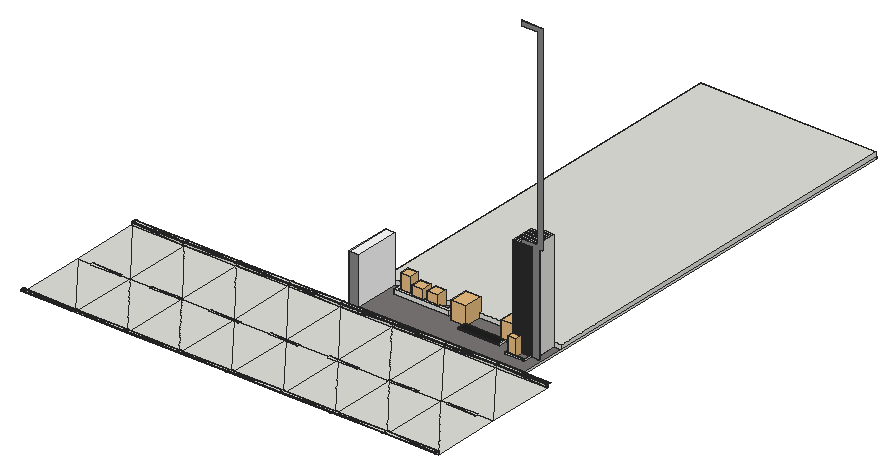
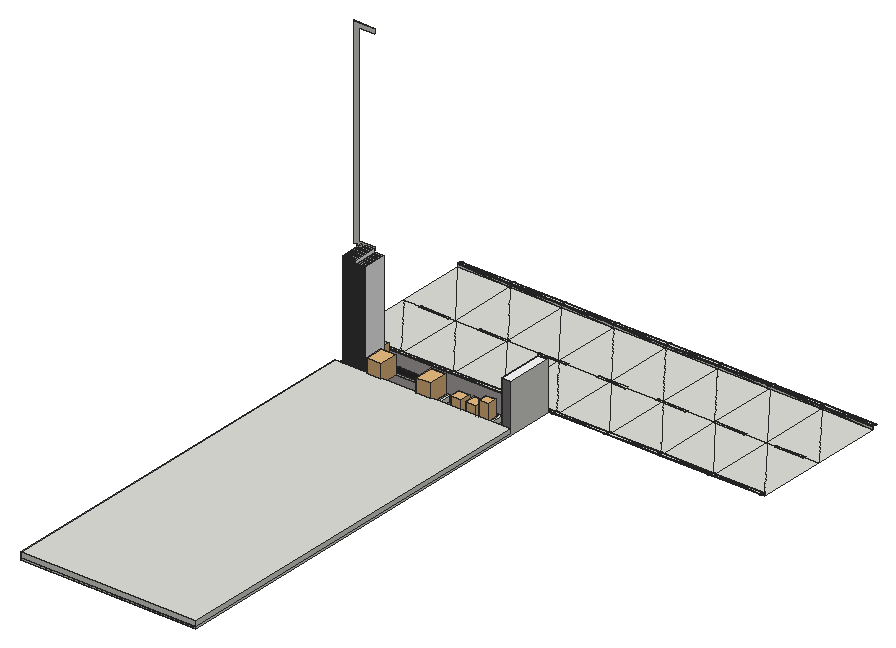
# SketchUp Ruby script. Lengths in inches.
U = 1.inch
M = Sketchup.active_model
def pt(a) = Geom::Point3d.new(a.map { |v| v * U })
def face(e, loops, mat)
  f = e.add_face(loops[0].map { |a| pt(a) })
  loops[1..].each { |l| e.add_face(l.map { |a| pt(a) }).erase! }
  f.material = f.back_material = mat if mat
  f
end
# faces: each face lists its corners as indices into pts; further lists are holes
def faces(e, pts, list, mat = nil) = list.each { |f| face(e, (f[0].is_a?(Array) ? f : [f]).map { |l| l.map { |i| pts[i] } }, mat) }
# xy, xz, yz: faces in a plane at the given z, y or x. An outline is a flat list of corners, or four numbers for a rectangle; further outlines are holes
def ring(l) = l.size == 4 ? [[l[0], l[1]], [l[2], l[1]], [l[2], l[3]], [l[0], l[3]]] : l.each_slice(2).to_a
def flat(e, list, mat, &to3) = list.each { |f| face(e, (f[0].is_a?(Array) ? f : [f]).map { |l| ring(l).map { |u, v| to3.(u, v) } }, mat) }
def xy(e, z, list, mat = nil) = flat(e, list, mat) { |x, y| [x, y, z] }
def xz(e, y, list, mat = nil) = flat(e, list, mat) { |x, z| [x, y, z] }
def yz(e, x, list, mat = nil) = flat(e, list, mat) { |y, z| [x, y, z] }
def lines(e, pts, list) = list.each { |a, b| e.add_line(pt(pts[a]), pt(pts[b])) }
# prism: a flat outline (further loops are holes) pulled along v
def prism(e, loops, v, mat = nil)
  f = face(e, loops, mat); d = Geom::Vector3d.new(v.map { |x| x * U })
  f.pushpull(f.normal.samedirection?(d) ? d.length : -d.length)
end
def box(e, o, s, mat = nil) = prism(e, [[o, [o[0] + s[0], o[1], o[2]], [o[0] + s[0], o[1] + s[1], o[2]], [o[0], o[1] + s[1], o[2]]]], [0, 0, s[2]], mat)
def at(x, y, z, deg = 0) = Geom::Transformation.translation(pt([x, y, z])) * Geom::Transformation.rotation(ORIGIN, Z_AXIS, deg.degrees)
def axes(o, x, y, z) = Geom::Transformation.new([*x, 0, *y, 0, *z, 0, *pt(o).to_a, 1])
def part(name) = M.definitions.add(name)
# library, detail: a bought-in or finely detailed component or shape, given as its bounding box
def library(name, o, s) = part(name).tap { |d| box(d.entities, o, s) }
def detail(e, o, s) = box(e.add_group.entities, o, s)
def put(e, d, t, mat = nil) = e.add_instance(d, t).tap { |i| i.material = mat if mat }
def group(e, t, mat = nil) = e.add_group.tap { |g| g.transformation = t; g.material = mat if mat }.entities
root = M.entities
M.materials.add("Marble White 602 38.29cm").color = [255, 255, 255]
M.materials.add("T8500 Silicone plaster D1 27.81cm").color = [255, 255, 255]
M.materials.add("Tiles B 130cm").color = [122, 119, 118]
M.materials.add("Tiles Marble Black 01 160cm").color = [32, 32, 32]
M.materials.add("Wall Paint Bumpy 01 Gray 100cm").color = [135, 135, 135]
M.materials.add("Wood Amboyan 13.2cm").color = [255, 255, 255]
c1 = library("Potted Plant 02",[-16.98,-19.78,0],[30.04,38.68,37.52])
c2 = library("Indoor Plant 004",[-26.75,-21.09,0],[44.44,41.03,87.36])
c3 = library("Potted Plant 50-12",[-6.11,-5.26,0],[11.24,10.56,13.41])
c4 = library("Sedum Plant 66-24",[-7.97,-7.95,0.04],[16.42,16.31,19.57])
c5 = library("Potted Plant 13",[-10,-7.28,0],[18.93,15.17,39.22])
c6 = part("Vertical panel \#2")
box(c6.entities,[0,-6.5625,0],[1.16,30,129.34],"Wood Amboyan 13.2cm")
c7 = part("Vertical panel \#1")
xy(c7.entities,0,[[0,-6.5625,1.16,23.4375]])
xy(c7.entities,125.9,[[0,-6.5625,1.16,23.4375]])
xz(c7.entities,-6.5625,[[0,0,1.16,125.9]],"Wood Amboyan 13.2cm")
xz(c7.entities,23.4375,[[0,0,1.16,125.9]])
yz(c7.entities,0,[[-6.5625,0,23.4375,125.9]])
yz(c7.entities,1.16,[[-6.5625,0,23.4375,125.9]])
c8 = part("Vertical panel \#3")
box(c8.entities,[0,-6.6875,0],[1.16,30.125,129.71],"Wood Amboyan 13.2cm")
c9 = part("Vertical panel \#4")
box(c9.entities,[0,-6.5625,0],[1.16,30,129.34],"Wood Amboyan 13.2cm")
c10 = part("Vertical panel \#5")
box(c10.entities,[0,-6.6875,0],[1.16,30.125,129.21],"Wood Amboyan 13.2cm")
c11 = part("Vertical panel \#6")
xy(c11.entities,0,[[0,0,1.16,23.4375]])
xy(c11.entities,129.21,[[0,0,1.16,23.4375]])
xz(c11.entities,0,[[0,0,1.16,129.21]],"Wood Amboyan 13.2cm")
xz(c11.entities,23.4375,[[0,0,1.16,129.21]])
yz(c11.entities,0,[[0,0,23.4375,129.21]])
yz(c11.entities,1.16,[[0,0,23.4375,129.21]])
c12 = part("Vertical panel \#7")
box(c12.entities,[0,-6.5625,0],[1.16,30,129.21])
c13 = part("Vertical panel assembly")
put(c13.entities,c9,at(0,0,0),"Wood Amboyan 13.2cm")
put(c13.entities,c10,at(2.58,0,0))
put(c13.entities,c11,at(5.16,0,0))
put(c13.entities,c12,at(7.75,0,0))
c14 = part("Component\#12")
xy(c14.entities,0,[[0,0,53.8125,10.8125]])
xy(c14.entities,1.8125,[[0,-0.5,2,0],[2,-0.5,51.8125,0],[51.8125,-0.5,53.8125,0]])
xy(c14.entities,2.125,[[51.8125,-0.5,53.8125,10.8125]])
xy(c14.entities,2.125,[[0,-0.5,2,10.8125]],"Marble White 602 38.29cm")
xy(c14.entities,2.125,[[2,-0.5,51.8125,10.8125]],"Tiles Marble Black 01 160cm")
xz(c14.entities,-0.5,[[0,1.8125,53.8125,2.125]],"Marble White 602 38.29cm")
xz(c14.entities,0,[[0,0,53.8125,1.8125]],"Tiles Marble Black 01 160cm")
xz(c14.entities,10.8125,[[0,0,53.8125,2.125]])
yz(c14.entities,0,[[0,0,0,1.8125,-0.5,1.8125,-0.5,2.125,10.8125,2.125,10.8125,0]])
yz(c14.entities,53.8125,[[0,0,10.8125,0,10.8125,2.125,-0.5,2.125,-0.5,1.8125,0,1.8125]])
xy(root,-10.11,[[0,4.875,66.91,4.875,0,92.46],[66.91,4.875,66.91,92.46,0,92.46],[133.82,4.875,133.82,92.46,66.91,92.46],[66.91,4.875,133.82,4.875,66.91,92.46],[133.82,4.875,200.73,4.875,133.82,92.46],
  [200.73,4.875,200.73,92.46,133.82,92.46],[200.73,4.875,267.64,4.875,200.73,92.46],[267.64,4.875,267.64,92.46,200.73,92.46],[267.64,4.875,334.55,4.875,267.64,92.46],[334.55,4.875,334.55,92.46,267.64,92.46],
  [334.55,4.875,401.46,4.875,334.55,92.46],[401.46,4.875,401.46,92.46,334.55,92.46],[401.46,4.875,468.37,4.875,401.46,92.46],[468.37,4.875,468.37,92.46,401.46,92.46],[468.37,4.875,535.28,4.875,468.37,92.46],
  [535.28,4.875,535.28,92.46,468.37,92.46],[0,92.46,66.91,92.46,0,180.06],[66.91,92.46,66.91,180.06,0,180.06],[133.82,92.46,133.82,180.06,66.91,180.06],[66.91,92.46,133.82,92.46,66.91,180.06],
  [133.82,92.46,200.73,92.46,133.82,180.06],[200.73,92.46,200.73,180.06,133.82,180.06],[200.73,92.46,267.64,92.46,200.73,180.06],[267.64,92.46,267.64,180.06,200.73,180.06],[267.64,92.46,334.55,92.46,267.64,180.06],
  [334.55,92.46,334.55,180.06,267.64,180.06],[334.55,92.46,401.46,92.46,334.55,180.06],[401.46,92.46,401.46,180.06,334.55,180.06],[401.46,92.46,468.37,92.46,401.46,180.06],[468.37,92.46,468.37,180.06,401.46,180.06],
  [468.37,92.46,535.28,92.46,468.37,180.06],[535.28,92.46,535.28,180.06,468.37,180.06]])
xy(root,-10.1,[[17.9,90.98,56.09,90.98,17.9,93.94],[56.09,90.98,56.09,93.94,17.9,93.94],[132.47,90.98,132.47,93.94,94.28,93.94],[94.28,90.98,132.47,90.98,94.28,93.94],[170.67,90.98,208.86,90.98,170.67,93.94],
  [208.86,90.98,208.86,93.94,170.67,93.94],[247.05,90.98,285.24,90.98,247.05,93.94],[285.24,90.98,285.24,93.94,247.05,93.94],[323.43,90.98,361.62,90.98,323.43,93.94],[361.62,90.98,361.62,93.94,323.43,93.94],
  [399.8125,90.98,438.01,90.98,399.8125,93.94],[438.01,90.98,438.01,93.94,399.8125,93.94],[476.2,90.98,514.39,90.98,476.2,93.94],[514.39,90.98,514.39,93.94,476.2,93.94]])
xy(root,-8.375,[[275.19,185.76,501.69,751.57]])
xy(root,-6,[[0,0.15,0.21,0.15,0,0.34],[0.21,0.15,0.21,0.34,0,0.34],[0.21,0.15,66.91,0.15,0.21,0.34],[66.91,0.15,66.91,0.34,0.21,0.34],[66.91,0.15,133.82,0.15,133.82,0.34],
  [66.91,0.15,133.82,0.34,66.91,0.34],[133.82,0.15,200.73,0.15,200.73,0.34],[133.82,0.15,200.73,0.34,133.82,0.34],[200.73,0.15,267.64,0.15,200.73,0.34],[267.64,0.15,267.64,0.34,200.73,0.34],
  [267.64,0.15,334.55,0.15,334.55,0.34],[267.64,0.15,334.55,0.34,267.64,0.34],[334.55,0.15,401.46,0.15,401.46,0.34],[334.55,0.15,401.46,0.34,334.55,0.34],[401.46,0.15,468.37,0.15,468.37,0.34],
  [401.46,0.15,468.37,0.34,401.46,0.34],[468.37,0.15,535.06,0.15,468.37,0.34],[535.06,0.15,535.06,0.34,468.37,0.34],[535.06,0.15,535.28,0.15,535.06,0.34],[535.28,0.15,535.28,0.34,535.06,0.34],
  [0,0.34,0.21,0.34,0,4.1],[0.21,0.34,0.21,4.1,0,4.1],[0.21,0.34,66.91,0.34,0.21,4.1],[66.91,0.34,66.91,4.1,0.21,4.1],[66.91,0.34,133.82,0.34,133.82,4.1],
  [66.91,0.34,133.82,4.1,66.91,4.1],[133.82,0.34,200.73,0.34,200.73,4.1],[133.82,0.34,200.73,4.1,133.82,4.1],[200.73,0.34,267.64,0.34,267.64,4.1],[200.73,0.34,267.64,4.1,200.73,4.1],
  [267.64,0.34,334.55,0.34,334.55,4.1],[267.64,0.34,334.55,4.1,267.64,4.1],[334.55,0.34,401.46,0.34,401.46,4.1],[334.55,0.34,401.46,4.1,334.55,4.1],[401.46,0.34,468.37,0.34,468.37,4.1],
  [401.46,0.34,468.37,4.1,401.46,4.1],[468.37,0.34,535.06,0.34,468.37,4.1],[535.06,0.34,535.06,4.1,468.37,4.1],[535.06,0.34,535.28,0.34,535.06,4.1],[535.28,0.34,535.28,4.1,535.06,4.1],
  [0,4.1,0.21,4.1,0,4.52],[0.21,4.1,0.21,4.52,0,4.52],[0.21,4.1,66.91,4.1,0.21,4.52],[66.91,4.1,66.91,4.52,0.21,4.52],[133.82,4.1,133.82,4.52,66.91,4.52],
  [66.91,4.1,133.82,4.1,66.91,4.52],[133.82,4.1,200.73,4.1,133.82,4.52],[200.73,4.1,200.73,4.52,133.82,4.52],[200.73,4.1,267.64,4.1,267.64,4.52],[200.73,4.1,267.64,4.52,200.73,4.52],
  [267.64,4.1,334.55,4.1,267.64,4.52],[334.55,4.1,334.55,4.52,267.64,4.52],[334.55,4.1,401.46,4.1,334.55,4.52],[401.46,4.1,401.46,4.52,334.55,4.52],[401.46,4.1,468.37,4.1,401.46,4.52],
  [468.37,4.1,468.37,4.52,401.46,4.52],[468.37,4.1,535.06,4.1,468.37,4.52],[535.06,4.1,535.06,4.52,468.37,4.52],[535.06,4.1,535.28,4.1,535.06,4.52],[535.28,4.1,535.28,4.52,535.06,4.52],
  [0,180.41,0.23,180.41,0,180.66],[0.23,180.41,0.23,180.66,0,180.66],[0.23,180.41,66.91,180.41,0.23,180.66],[66.91,180.41,66.91,180.66,0.23,180.66],[66.91,180.41,133.82,180.41,133.82,180.66],
  [66.91,180.41,133.82,180.66,66.91,180.66],[133.82,180.41,200.73,180.41,200.73,180.66],[133.82,180.41,200.73,180.66,133.82,180.66],[200.73,180.41,267.64,180.41,200.73,180.66],[267.64,180.41,267.64,180.66,200.73,180.66],
  [267.64,180.41,334.55,180.41,334.55,180.66],[267.64,180.41,334.55,180.66,267.64,180.66],[334.55,180.41,401.46,180.41,401.46,180.66],[334.55,180.41,401.46,180.66,334.55,180.66],[401.46,180.41,468.37,180.41,468.37,180.66],
  [401.46,180.41,468.37,180.66,401.46,180.66],[468.37,180.41,535.01,180.41,468.37,180.66],[535.01,180.41,535.01,180.66,468.37,180.66],[535.01,180.41,535.28,180.41,535.01,180.66],[535.28,180.41,535.28,180.66,535.01,180.66],
  [0,180.66,0.23,180.66,0,184.49],[0.23,180.66,0.23,184.49,0,184.49],[0.23,180.66,66.91,180.66,0.23,184.49],[66.91,180.66,66.91,184.49,0.23,184.49],[66.91,180.66,133.82,180.66,133.82,184.49],
  [66.91,180.66,133.82,184.49,66.91,184.49],[133.82,180.66,200.73,180.66,200.73,184.49],[133.82,180.66,200.73,184.49,133.82,184.49],[200.73,180.66,267.64,180.66,267.64,184.49],[200.73,180.66,267.64,184.49,200.73,184.49],
  [267.64,180.66,334.55,180.66,334.55,184.49],[267.64,180.66,334.55,184.49,267.64,184.49],[334.55,180.66,401.46,180.66,401.46,184.49],[334.55,180.66,401.46,184.49,334.55,184.49],[401.46,180.66,468.37,180.66,468.37,184.49],
  [401.46,180.66,468.37,184.49,401.46,184.49],[468.37,180.66,535.01,180.66,468.37,184.49],[535.01,180.66,535.01,184.49,468.37,184.49],[535.01,180.66,535.28,180.66,535.01,184.49],[535.28,180.66,535.28,184.49,535.01,184.49],
  [0,184.49,0.23,184.49,0,184.78],[0.23,184.49,0.23,184.78,0,184.78],[0.23,184.49,66.91,184.49,0.23,184.78],[66.91,184.49,66.91,184.78,0.23,184.78],[133.82,184.49,133.82,184.78,66.91,184.78],
  [66.91,184.49,133.82,184.49,66.91,184.78],[133.82,184.49,200.73,184.49,133.82,184.78],[200.73,184.49,200.73,184.78,133.82,184.78],[200.73,184.49,267.64,184.49,267.64,184.78],[200.73,184.49,267.64,184.78,200.73,184.78],
  [267.64,184.49,334.55,184.49,267.64,184.78],[334.55,184.49,334.55,184.78,267.64,184.78],[334.55,184.49,401.46,184.49,334.55,184.78],[401.46,184.49,401.46,184.78,334.55,184.78],[401.46,184.49,468.37,184.49,401.46,184.78],
  [468.37,184.49,468.37,184.78,401.46,184.78],[468.37,184.49,535.01,184.49,468.37,184.78],[535.01,184.49,535.01,184.78,468.37,184.78],[535.01,184.49,535.28,184.49,535.01,184.78],[535.28,184.49,535.28,184.78,535.01,184.78]])
xy(root,-6,[[[287.19,185.76,501.69,185.76,501.69,751.57,275.19,751.57,275.19,244.57,287.19,244.57],[297.97,228.57,297.97,244.57,301.97,244.57,301.97,232.57,365.1,232.57,365.1,244.57,369.1,244.57,369.1,228.57]]],"Tiles B 130cm")
xy(root,-5.9,[[462.69,202.57,462.69,214.57,463.69,214.57,463.69,203.57,486.92,203.57,486.92,213.79,487.92,213.79,487.92,202.57],[487.92,213.79,497.86,214.57],[475.6,214.57,476.76,244.57]])
xy(root,-0.4375,[[297.97,228.57,369.1,228.57,369.1,244.57,365.1,244.57,365.1,232.57,301.97,232.57,301.97,244.57,297.97,244.57]])
xy(root,54,[[275.19,185.76,287.19,244.57]],"T8500 Silicone plaster D1 27.81cm")
xz(root,0,[[0,-6.69,0.21,-6.69,0,-6.26],[0.21,-6.69,0.21,-6.26,0,-6.26],[0.21,-6.69,66.91,-6.69,0.21,-6.26],[66.91,-6.69,66.91,-6.26,0.21,-6.26],[66.91,-6.69,133.82,-6.26,66.91,-6.26],
  [66.91,-6.69,133.82,-6.69,133.82,-6.26],[133.82,-6.69,200.73,-6.26,133.82,-6.26],[133.82,-6.69,200.73,-6.69,200.73,-6.26],[200.73,-6.69,267.64,-6.26,200.73,-6.26],[200.73,-6.69,267.64,-6.69,267.64,-6.26],
  [267.64,-6.69,334.55,-6.26,267.64,-6.26],[267.64,-6.69,334.55,-6.69,334.55,-6.26],[334.55,-6.69,401.46,-6.26,334.55,-6.26],[334.55,-6.69,401.46,-6.69,401.46,-6.26],[401.46,-6.69,468.37,-6.26,401.46,-6.26],
  [401.46,-6.69,468.37,-6.69,468.37,-6.26],[468.37,-6.69,535.06,-6.69,468.37,-6.26],[535.06,-6.69,535.06,-6.26,468.37,-6.26],[535.06,-6.69,535.28,-6.69,535.06,-6.26],[535.28,-6.69,535.28,-6.26,535.06,-6.26]])
xz(root,4.875,[[0,-10.11,0,-6.93,0.21,-6.93],[0,-10.11,0.21,-6.93,0.21,-10.11],[0.21,-10.11,0.21,-6.93,66.91,-6.93],[0.21,-10.11,66.91,-6.93,66.91,-10.11],[66.91,-10.11,133.82,-6.93,133.82,-10.11],
  [66.91,-10.11,66.91,-6.93,133.82,-6.93],[133.82,-10.11,133.82,-6.93,200.73,-6.93],[133.82,-10.11,200.73,-6.93,200.73,-10.11],[200.73,-10.11,200.73,-6.93,267.64,-10.11],[267.64,-10.11,200.73,-6.93,267.64,-6.93],
  [267.64,-10.11,267.64,-6.93,334.55,-6.93],[267.64,-10.11,334.55,-6.93,334.55,-10.11],[334.55,-10.11,334.55,-6.93,401.46,-6.93],[334.55,-10.11,401.46,-6.93,401.46,-10.11],[401.46,-10.11,401.46,-6.93,468.37,-6.93],
  [401.46,-10.11,468.37,-6.93,468.37,-10.11],[468.37,-10.11,468.37,-6.93,535.06,-6.93],[468.37,-10.11,535.06,-6.93,535.06,-10.11],[535.06,-10.11,535.06,-6.93,535.28,-6.93],[535.06,-10.11,535.28,-6.93,535.28,-10.11],
  [0,-6.93,0,-6.49,0.21,-6.49],[0,-6.93,0.21,-6.49,0.21,-6.93],[0.21,-6.93,0.21,-6.49,66.91,-6.49],[0.21,-6.93,66.91,-6.49,66.91,-6.93],[133.82,-6.93,66.91,-6.49,133.82,-6.49],
  [66.91,-6.93,66.91,-6.49,133.82,-6.93],[133.82,-6.93,133.82,-6.49,200.73,-6.93],[200.73,-6.93,133.82,-6.49,200.73,-6.49],[200.73,-6.93,200.73,-6.49,267.64,-6.49],[200.73,-6.93,267.64,-6.49,267.64,-6.93],
  [267.64,-6.93,267.64,-6.49,334.55,-6.93],[334.55,-6.93,267.64,-6.49,334.55,-6.49],[334.55,-6.93,334.55,-6.49,401.46,-6.93],[401.46,-6.93,334.55,-6.49,401.46,-6.49],[401.46,-6.93,401.46,-6.49,468.37,-6.93],
  [468.37,-6.93,401.46,-6.49,468.37,-6.49],[468.37,-6.93,468.37,-6.49,535.06,-6.49],[468.37,-6.93,535.06,-6.49,535.06,-6.93],[535.06,-6.93,535.06,-6.49,535.28,-6.49],[535.06,-6.93,535.28,-6.49,535.28,-6.93]])
xz(root,180.06,[[0,-10.11,0.23,-10.11,0,-7.19],[0.23,-10.11,0.23,-7.19,0,-7.19],[0.23,-10.11,66.91,-10.11,0.23,-7.19],[66.91,-10.11,66.91,-7.19,0.23,-7.19],[66.91,-10.11,133.82,-10.11,133.82,-7.19],
  [66.91,-10.11,133.82,-7.19,66.91,-7.19],[133.82,-10.11,200.73,-10.11,200.73,-7.19],[133.82,-10.11,200.73,-7.19,133.82,-7.19],[200.73,-10.11,267.64,-10.11,200.73,-7.19],[267.64,-10.11,267.64,-7.19,200.73,-7.19],
  [267.64,-10.11,334.55,-10.11,334.55,-7.19],[267.64,-10.11,334.55,-7.19,267.64,-7.19],[334.55,-10.11,401.46,-10.11,401.46,-7.19],[334.55,-10.11,401.46,-7.19,334.55,-7.19],[401.46,-10.11,468.37,-10.11,468.37,-7.19],
  [401.46,-10.11,468.37,-7.19,401.46,-7.19],[468.37,-10.11,535.01,-10.11,468.37,-7.19],[535.01,-10.11,535.01,-7.19,468.37,-7.19],[535.01,-10.11,535.28,-10.11,535.01,-7.19],[535.28,-10.11,535.28,-7.19,535.01,-7.19],
  [0,-7.19,0.23,-7.19,0,-6.49],[0.23,-7.19,0.23,-6.49,0,-6.49],[0.23,-7.19,66.91,-7.19,0.23,-6.49],[66.91,-7.19,66.91,-6.49,0.23,-6.49],[133.82,-7.19,133.82,-6.49,66.91,-6.49],
  [66.91,-7.19,133.82,-7.19,66.91,-6.49],[133.82,-7.19,200.73,-7.19,133.82,-6.49],[200.73,-7.19,200.73,-6.49,133.82,-6.49],[200.73,-7.19,267.64,-6.49,200.73,-6.49],[200.73,-7.19,267.64,-7.19,267.64,-6.49],
  [267.64,-7.19,334.55,-7.19,267.64,-6.49],[334.55,-7.19,334.55,-6.49,267.64,-6.49],[334.55,-7.19,401.46,-7.19,334.55,-6.49],[401.46,-7.19,401.46,-6.49,334.55,-6.49],[401.46,-7.19,468.37,-7.19,401.46,-6.49],
  [468.37,-7.19,468.37,-6.49,401.46,-6.49],[468.37,-7.19,535.01,-7.19,468.37,-6.49],[535.01,-7.19,535.01,-6.49,468.37,-6.49],[535.01,-7.19,535.28,-7.19,535.01,-6.49],[535.28,-7.19,535.28,-6.49,535.01,-6.49]])
xz(root,184.93,[[0,-6.75,0,-6.26,0.23,-6.26],[0,-6.75,0.23,-6.26,0.23,-6.75],[0.23,-6.75,0.23,-6.26,66.91,-6.26],[0.23,-6.75,66.91,-6.26,66.91,-6.75],[133.82,-6.75,66.91,-6.26,133.82,-6.26],
  [66.91,-6.75,66.91,-6.26,133.82,-6.75],[133.82,-6.75,133.82,-6.26,200.73,-6.75],[200.73,-6.75,133.82,-6.26,200.73,-6.26],[200.73,-6.75,200.73,-6.26,267.64,-6.75],[267.64,-6.75,200.73,-6.26,267.64,-6.26],
  [267.64,-6.75,267.64,-6.26,334.55,-6.75],[334.55,-6.75,267.64,-6.26,334.55,-6.26],[334.55,-6.75,334.55,-6.26,401.46,-6.75],[401.46,-6.75,334.55,-6.26,401.46,-6.26],[401.46,-6.75,401.46,-6.26,468.37,-6.75],
  [468.37,-6.75,401.46,-6.26,468.37,-6.26],[468.37,-6.75,468.37,-6.26,535.01,-6.26],[468.37,-6.75,535.01,-6.26,535.01,-6.75],[535.01,-6.75,535.01,-6.26,535.28,-6.26],[535.01,-6.75,535.28,-6.26,535.28,-6.75]])
xz(root,185.76,[[275.19,-8.375,501.69,-8.375,501.69,-6,287.19,-6,287.19,54,275.19,54]],"Wall Paint Bumpy 01 Gray 100cm")
xz(root,202.57,[[462.69,-5.9,487.92,-3.9]])
xz(root,203.57,[[463.69,-5.9,486.92,-3.9]])
xz(root,213.79,[[486.92,-5.9,487.92,-3.9]])
xz(root,213.79,[[487.92,-5.9,497.86,-5.9,497.86,121.5,501.69,121.5,501.69,378,474.63,378,474.63,372,495.69,372,495.69,125.96,474.63,125.96,474.63,121.5,487.92,121.5]],"Wall Paint Bumpy 01 Gray 100cm")
xz(root,214.57,[[462.69,-5.9,463.69,-3.9],[487.92,-5.9,487.92,121.5,476.76,121.5,476.76,123.3125,475.6,123.3125,475.6,121.5,474.63,121.5,474.63,125.96,495.69,125.96,495.69,372,474.63,372,474.63,378,501.69,378,501.69,121.5,497.86,121.5,497.86,-5.9]])
xz(root,214.57,[[475.6,-5.9,476.76,121.5]],"Wood Amboyan 13.2cm")
xz(root,228.57,[[297.97,-6,369.1,-0.4375]])
xz(root,232.57,[[301.97,-6,365.1,-0.4375]])
xz(root,244.57,[[297.97,-6,301.97,-0.4375],[365.1,-6,369.1,-0.4375],[475.6,-5.9,476.76,123.3125]])
xz(root,244.57,[[275.19,-6,287.19,54]],"Tiles B 130cm")
xz(root,751.57,[[275.19,-8.375,501.69,-6]])
yz(root,275.19,[[185.76,-8.375,185.76,54,244.57,54,244.57,-6,751.57,-6,751.57,-8.375]])
yz(root,287.19,[[185.76,-6,244.57,54]],"T8500 Silicone plaster D1 27.81cm")
yz(root,297.97,[[228.57,-6,244.57,-0.4375]])
yz(root,301.97,[[232.57,-6,244.57,-0.4375]])
yz(root,365.1,[[232.57,-6,244.57,-0.4375]])
yz(root,369.1,[[228.57,-6,244.57,-0.4375]])
yz(root,462.69,[[202.57,-5.9,214.57,-3.9]])
yz(root,463.69,[[203.57,-5.9,214.57,-3.9]])
yz(root,475.6,[[214.57,-5.9,244.57,123.3125]],"Wood Amboyan 13.2cm")
yz(root,476.76,[[214.57,-5.9,244.57,123.3125]],"Wood Amboyan 13.2cm")
yz(root,486.92,[[203.57,-5.9,213.79,-3.9]])
yz(root,487.92,[[202.57,-5.9,213.79,-3.9],[213.79,-5.9,214.57,121.5]])
yz(root,497.86,[[213.79,-5.9,214.57,121.5]])
yz(root,501.69,[[185.76,-8.375,751.57,-6]])
p = [[0,4.875,-6.49],[0,4.79,-6.125],[0.21,4.79,-6.125],[0.21,4.875,-6.49],[66.91,4.875,-6.49],[66.91,4.79,-6.125],
  [133.82,4.79,-6.125],[133.82,4.875,-6.49],[200.73,4.79,-6.125],[200.73,4.875,-6.49],[267.64,4.79,-6.125],[267.64,4.875,-6.49],
  [334.55,4.79,-6.125],[334.55,4.875,-6.49],[401.46,4.79,-6.125],[401.46,4.875,-6.49],[468.37,4.79,-6.125],[468.37,4.875,-6.49],
  [535.06,4.79,-6.125],[535.06,4.875,-6.49],[535.28,4.79,-6.125],[535.28,4.875,-6.49],[0,180.14,-6.12],[0,180.06,-6.49],
  [0.23,180.06,-6.49],[0.23,180.14,-6.12],[66.91,180.06,-6.49],[66.91,180.14,-6.12],[133.82,180.06,-6.49],[133.82,180.14,-6.12],
  [200.73,180.06,-6.49],[200.73,180.14,-6.12],[267.64,180.06,-6.49],[267.64,180.14,-6.12],[334.55,180.06,-6.49],[334.55,180.14,-6.12],
  [401.46,180.06,-6.49],[401.46,180.14,-6.12],[468.37,180.06,-6.49],[468.37,180.14,-6.12],[535.01,180.14,-6.12],[535.01,180.06,-6.49],
  [535.28,180.06,-6.49],[535.28,180.14,-6.12],[0,0.15,-6],[0,0,-6.26],[0.21,0,-6.26],[0.21,0.15,-6],
  [66.91,0,-6.26],[66.91,0.15,-6],[133.82,0,-6.26],[133.82,0.15,-6],[200.73,0,-6.26],[200.73,0.15,-6],
  [267.64,0,-6.26],[267.64,0.15,-6],[334.55,0,-6.26],[334.55,0.15,-6],[401.46,0,-6.26],[401.46,0.15,-6],
  [468.37,0,-6.26],[468.37,0.15,-6],[535.06,0,-6.26],[535.06,0.15,-6],[535.28,0,-6.26],[535.28,0.15,-6],
  [0,184.93,-6.26],[0,184.78,-6],[0.23,184.78,-6],[0.23,184.93,-6.26],[66.91,184.78,-6],[66.91,184.93,-6.26],
  [133.82,184.78,-6],[133.82,184.93,-6.26],[200.73,184.78,-6],[200.73,184.93,-6.26],[267.64,184.78,-6],[267.64,184.93,-6.26],
  [334.55,184.78,-6],[334.55,184.93,-6.26],[401.46,184.78,-6],[401.46,184.93,-6.26],[468.37,184.78,-6],[468.37,184.93,-6.26],
  [535.01,184.78,-6],[535.01,184.93,-6.26],[535.28,184.78,-6],[535.28,184.93,-6.26],[0,4.52,-6],[0.21,4.52,-6],
  [66.91,4.52,-6],[133.82,4.52,-6],[200.73,4.52,-6],[267.64,4.52,-6],[334.55,4.52,-6],[401.46,4.52,-6],
  [468.37,4.52,-6],[535.06,4.52,-6],[535.28,4.52,-6],[0.23,180.41,-6],[0,180.41,-6],[66.91,180.41,-6],
  [133.82,180.41,-6],[200.73,180.41,-6],[267.64,180.41,-6],[334.55,180.41,-6],[401.46,180.41,-6],[468.37,180.41,-6],
  [535.01,180.41,-6],[535.28,180.41,-6]]
faces(root,p,[[0,1,2],[2,3,0],[4,3,2],[2,5,4],[4,5,6],[6,7,4],[8,9,7],[7,6,8],
  [9,8,10],[10,11,9],[11,10,12],[12,13,11],[14,15,13],[13,12,14],[16,17,15],[15,14,16],
  [18,19,17],[17,16,18],[20,21,19],[19,18,20],[22,23,24],[24,25,22],[26,27,25],[25,24,26],
  [28,29,27],[27,26,28],[29,28,30],[30,31,29],[32,33,31],[31,30,32],[34,35,33],[33,32,34],
  [35,34,36],[36,37,35],[37,36,38],[38,39,37],[40,39,38],[38,41,40],[42,43,40],[40,41,42],
  [44,45,46],[46,47,44],[48,49,47],[47,46,48],[49,48,50],[50,51,49],[51,50,52],[52,53,51],
  [53,52,54],[54,55,53],[56,57,55],[55,54,56],[58,59,57],[57,56,58],[60,61,59],[59,58,60],
  [60,62,63],[63,61,60],[63,62,64],[64,65,63],[66,67,68],[68,69,66],[70,71,69],[69,68,70],
  [72,73,71],[71,70,72],[74,75,73],[73,72,74],[75,74,76],[76,77,75],[78,79,77],[77,76,78],
  [79,78,80],[80,81,79],[81,80,82],[82,83,81],[84,85,83],[83,82,84],[86,87,85],[85,84,86],
  [1,88,89],[89,2,1],[89,90,5],[5,2,89],[5,90,91],[91,6,5],[92,8,6],[6,91,92],
  [93,10,8],[8,92,93],[10,93,94],[94,12,10],[12,94,95],[95,14,12],[96,16,14],[14,95,96],
  [97,18,16],[16,96,97],[18,97,98],[98,20,18],[25,99,100],[100,22,25],[99,25,27],[27,101,99],
  [101,27,29],[29,102,101],[102,29,31],[31,103,102],[103,31,33],[33,104,103],[35,105,104],[104,33,35],
  [37,106,105],[105,35,37],[39,107,106],[106,37,39],[39,40,108],[108,107,39],[43,109,108],[108,40,43]])
put(root,c1,axes([451.84,234.72,-6],[0.62,0,0],[0,0.62,0],[0,0,0.62]))
put(root,c1,axes([387.65,234.72,-6],[0.62,0,0],[0,0.62,0],[0,0,0.62]))
put(root,c2,axes([311.21,238.99,-6],[0.28,0,0],[0,0.28,0],[0,0,0.28]))
put(root,c3,axes([346.6875,238.01,-6],[1.24,0,0],[0,1.24,0],[0,0,1.24]))
g1 = group(root,at(275.19,244.57,-6))
box(g1,[0,0,0],[226.5,507,6])
g2 = group(root,at(462.69,221.14,-6))
box(g2,[0,0,0],[29.5625,23.4375,0.1])
put(root,c4,axes([326.49,237.55,-6.03],[0.84,0,0],[0,0.84,0],[0,0,0.84]))
put(root,c5,axes([469.65,208.19,-6],[0.53,0,0],[0,0.53,0],[0,0,0.53]))
put(root,c6,at(478.19,221.14,-5.9))
put(root,c7,at(462.69,221.14,-5.9),"Wood Amboyan 13.2cm")
put(root,c8,at(480.77,221.14,-5.9))
put(root,c13,at(483.35,221.14,-5.9))
put(root,c7,at(470.4375,221.14,-5.9),"Wood Amboyan 13.2cm")
put(root,c7,at(473.02,221.14,-5.9))
put(root,c7,at(465.27,221.14,-5.9),"Wood Amboyan 13.2cm")
put(root,c7,at(467.86,221.14,-5.9),"Wood Amboyan 13.2cm")
put(root,c14,at(393.8,212.14,-5.875))
